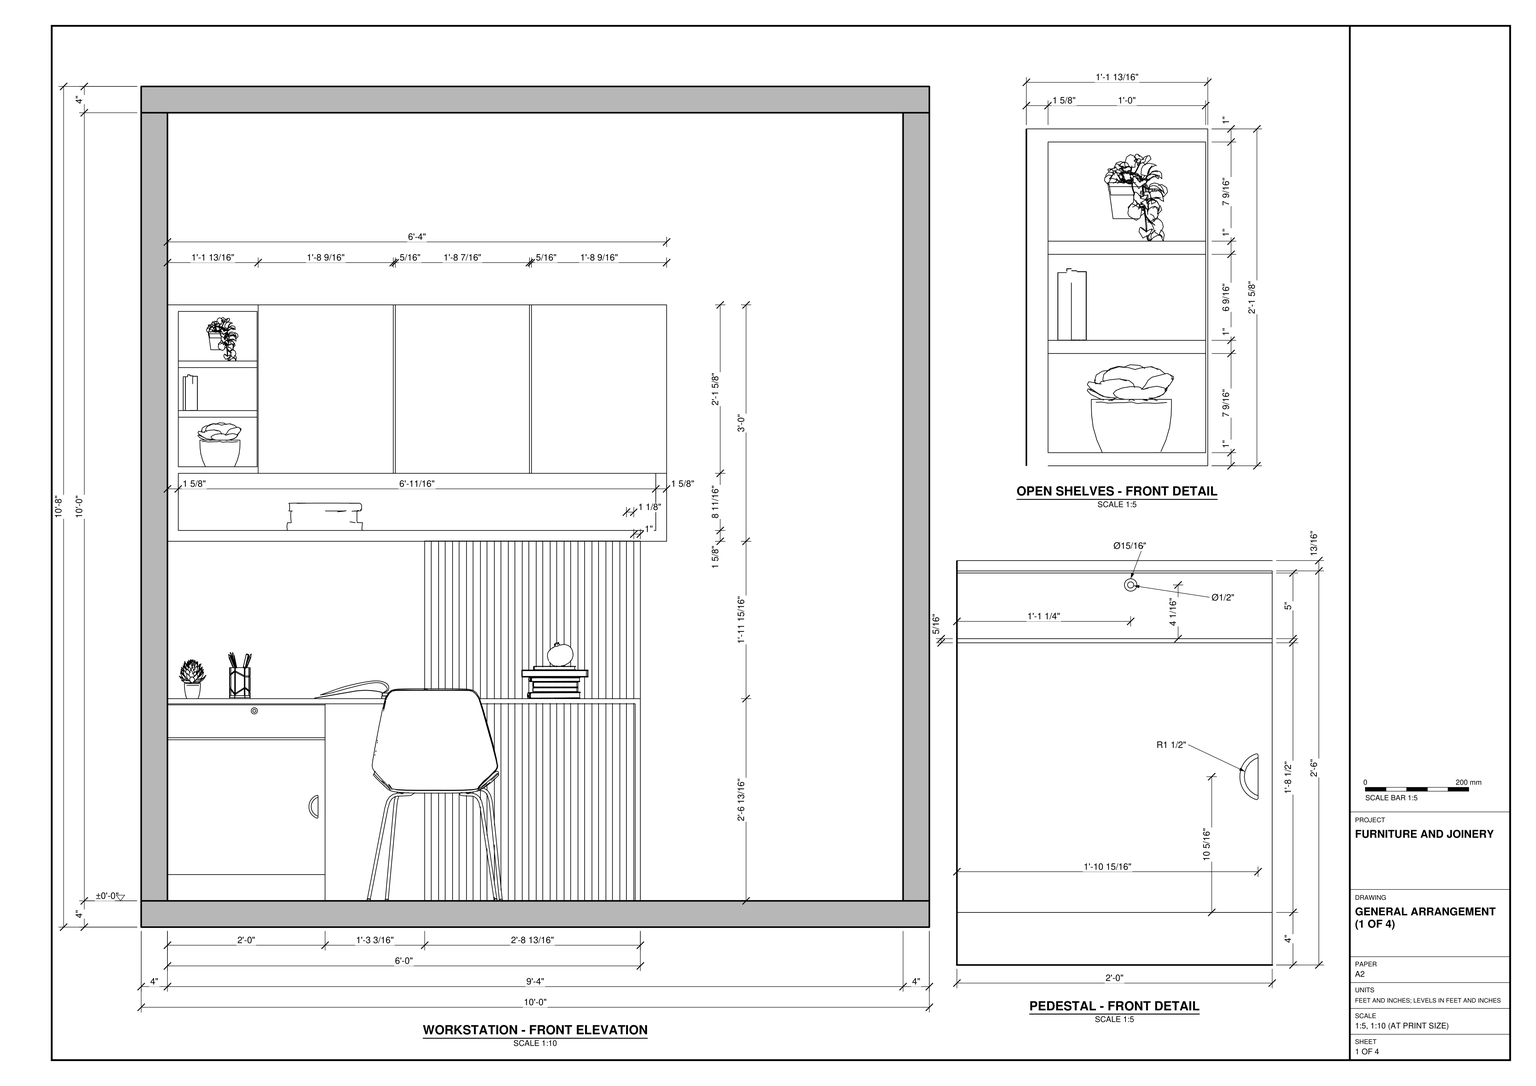
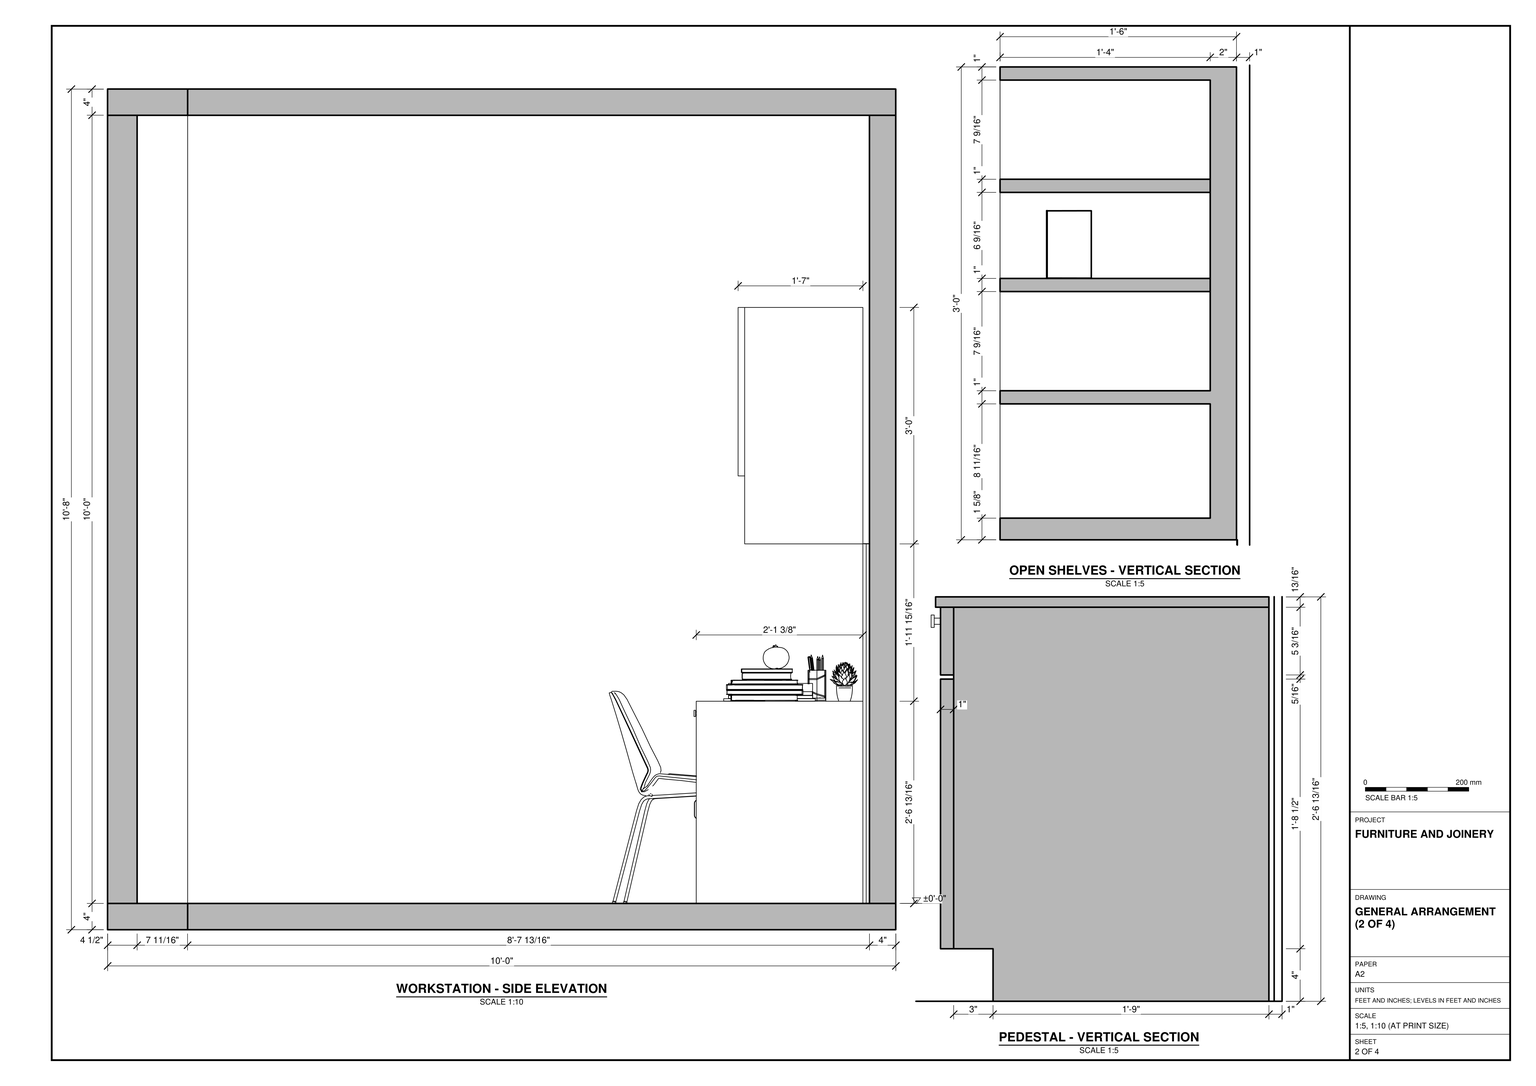
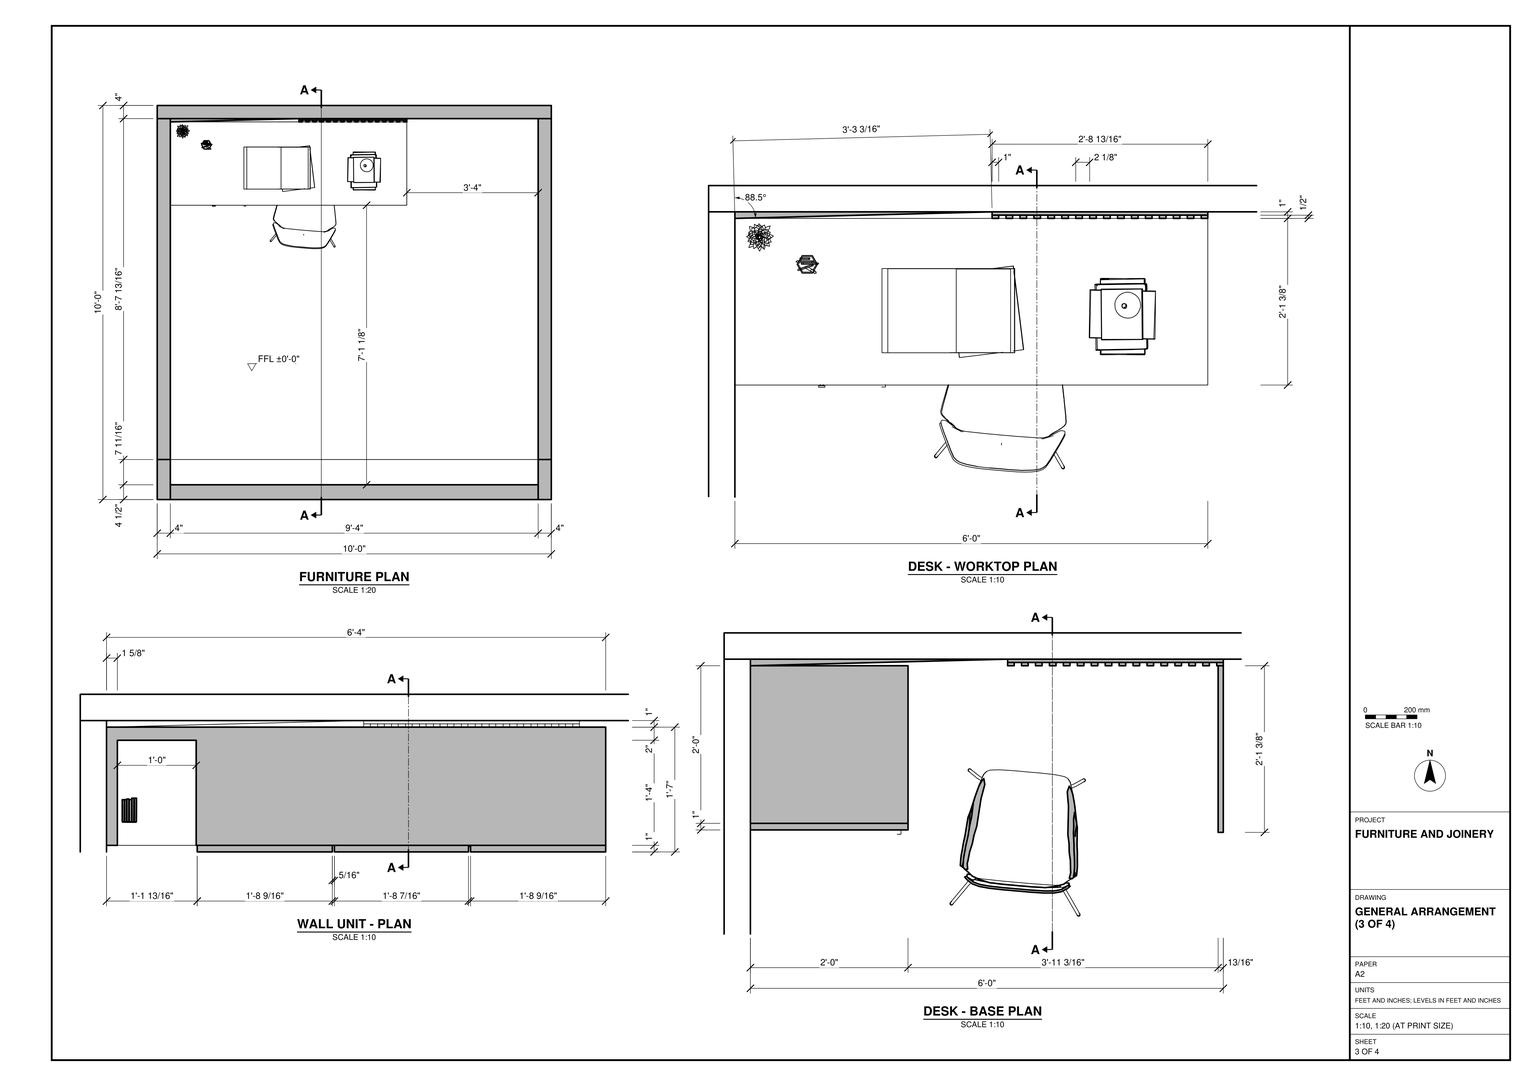
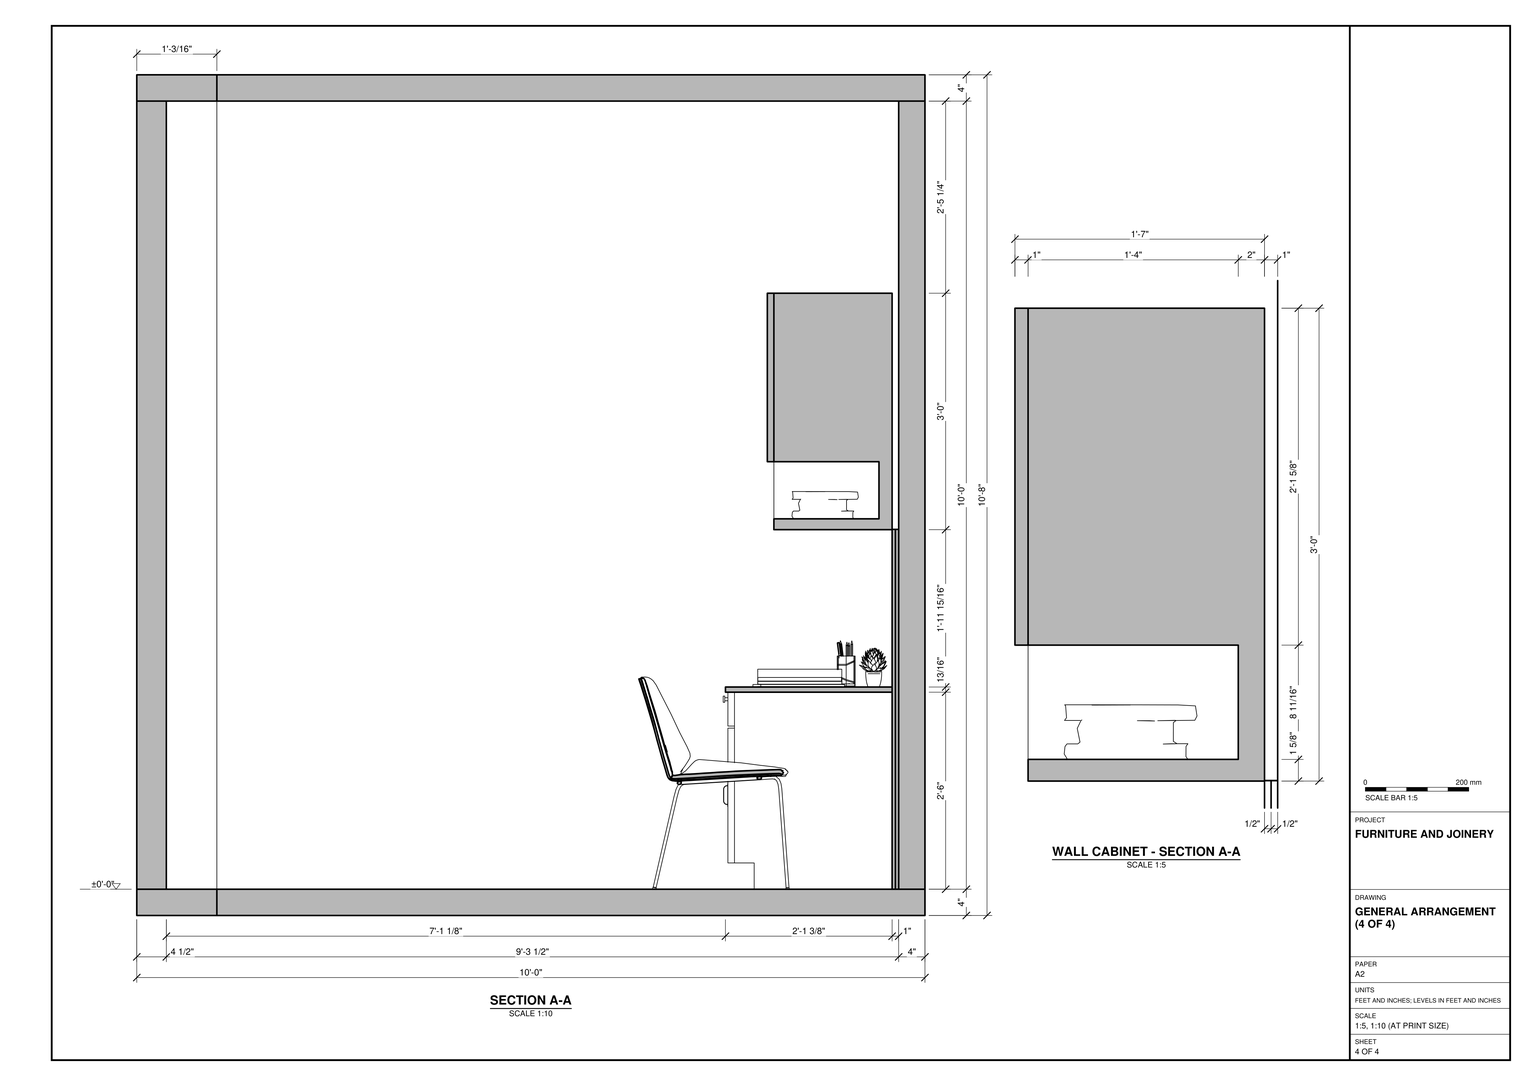
Build the workstation and its room shell in SketchUp from task_files/diagram_01.pdf. Work in feet and inches. The shell measures 10'-0" by 10'-0" in plan and 10'-8" in overall height. Use ±0'-0" as the finished floor level. Follow the wall thicknesses in plan and the floor and ceiling slab thicknesses in elevation.

Fit the desk against the back wall, starting at the left wall and leaving the space shown to its right. Model the continuous worktop, left storage pedestal and thin right end panel. Give the pedestal a shallow drawer above a cupboard door, with the pulls and recessed base shown in the details. Run the vertical slatted backing behind the right portion of the desk, from the floor to the underside of the wall unit. Above the desk, model the narrow stack of open cubbies on the left, the three cabinet fronts to their right and the continuous open shelf below. Place the chair facing the worktop in the knee space.

Decor and loose items such as the plants, books and pencil holders may be any suitable library components. Keep the shell elements and each furniture or joinery piece in separate groups or components, and use components for repeated parts. Save one SketchUp model as output_files/built_in_workstation_with_a_desk_and_wall_storage.skp.

# SketchUp Ruby script. Lengths in inches.
U = 1.inch
M = Sketchup.active_model
def pt(a) = Geom::Point3d.new(a.map { |v| v * U })
def face(e, loops, mat)
  f = e.add_face(loops[0].map { |a| pt(a) })
  loops[1..].each { |l| e.add_face(l.map { |a| pt(a) }).erase! }
  f.material = f.back_material = mat if mat
  f
end
# faces: each face lists its corners as indices into pts; further lists are holes
def faces(e, pts, list, mat = nil) = list.each { |f| face(e, (f[0].is_a?(Array) ? f : [f]).map { |l| l.map { |i| pts[i] } }, mat) }
# xy, xz, yz: faces in a plane at the given z, y or x. An outline is a flat list of corners, or four numbers for a rectangle; further outlines are holes
def ring(l) = l.size == 4 ? [[l[0], l[1]], [l[2], l[1]], [l[2], l[3]], [l[0], l[3]]] : l.each_slice(2).to_a
def flat(e, list, mat, &to3) = list.each { |f| face(e, (f[0].is_a?(Array) ? f : [f]).map { |l| ring(l).map { |u, v| to3.(u, v) } }, mat) }
def xy(e, z, list, mat = nil) = flat(e, list, mat) { |x, y| [x, y, z] }
def xz(e, y, list, mat = nil) = flat(e, list, mat) { |x, z| [x, y, z] }
def yz(e, x, list, mat = nil) = flat(e, list, mat) { |y, z| [x, y, z] }
def lines(e, pts, list) = list.each { |a, b| e.add_line(pt(pts[a]), pt(pts[b])) }
# prism: a flat outline (further loops are holes) pulled along v
def prism(e, loops, v, mat = nil)
  f = face(e, loops, mat); d = Geom::Vector3d.new(v.map { |x| x * U })
  f.pushpull(f.normal.samedirection?(d) ? d.length : -d.length)
end
def box(e, o, s, mat = nil) = prism(e, [[o, [o[0] + s[0], o[1], o[2]], [o[0] + s[0], o[1] + s[1], o[2]], [o[0], o[1] + s[1], o[2]]]], [0, 0, s[2]], mat)
def at(x, y, z, deg = 0) = Geom::Transformation.translation(pt([x, y, z])) * Geom::Transformation.rotation(ORIGIN, Z_AXIS, deg.degrees)
def axes(o, x, y, z) = Geom::Transformation.new([*x, 0, *y, 0, *z, 0, *pt(o).to_a, 1])
def part(name) = M.definitions.add(name)
# library, detail: a bought-in or finely detailed component or shape, given as its bounding box
def library(name, o, s) = part(name).tap { |d| box(d.entities, o, s) }
def detail(e, o, s) = box(e.add_group.entities, o, s)
def put(e, d, t, mat = nil) = e.add_instance(d, t).tap { |i| i.material = mat if mat }
def group(e, t, mat = nil) = e.add_group.tap { |g| g.transformation = t; g.material = mat if mat }.entities
root = M.entities
M.materials.add("Carpaint White 004 1.79cm").color = [255, 255, 255]
M.materials.add("Tiles Simple 01 100cm").color = [188, 184, 182]
M.materials.add("Wall Paint Olive Satin 300cm").color = [133, 140, 86]
M.materials.add("Wood Teak 33-35 100cm\#1").color = [135, 81, 33]
M.materials.add("XPS Yellow SSS 1.51cm").color = [255, 255, 255]
M.materials.add("[Color M09]4").color = [0, 0, 0]
c1 = library("Handle_25.skp\#1",[-1.74,-0.67,0],[3.48,0.67,1.38])
c2 = library("Potted Plant 50-24",[-2.18,-2.1,0],[4.36,4.2,6.7])
c3 = library("Potted Plant 50-23",[-3.4,-3.5,0],[6.8,7,9.93])
c4 = library("Books 53-17",[-2.19,-3.6875,0],[4.38,7.37,10.99])
c5 = library("Books 274 007",[-5.76,-5.0625,0],[11.51,10.11,4.16])
c6 = library("Chair 035",[-9.96,-11.17,0],[19.92,22.29,32.3125])
c7 = library("Plant 260 031 02",[-5.66,-10.61,-5.67],[17.04,23.05,21.91])
c8 = part("Group64\#1")
p = [[0,0,0],[0,0,-12.26],[-5.84,0,-12.26],[38,-1.69,0],[-38,-1.69,0],[38,1.69,0],
  [38,0,0],[-38,1.69,0],[5.84,0,-12.26],[-38,0,0],[0,0,-19.85]]
lines(c8.entities,p,[[0,1],[1,2],[3,4],[5,6],[7,5],[1,8],[9,0],[0,6],[8,10],[4,9],[6,3],[2,10],
  [9,7]])
c9 = part("Rectangle Light")
put(c9.entities,c8,at(0,0,0))
c10 = part("Group\#1")
xy(c10.entities,0,[[0,0,120,120]])
xy(c10.entities,4,[[0,0,120,120]],"Tiles Simple 01 100cm")
xz(c10.entities,0,[[0,0,120,4]])
xz(c10.entities,120,[[0,0,120,4]])
yz(c10.entities,0,[[0,0,120,4]])
yz(c10.entities,120,[[0,0,120,4]])
c11 = part("Group\#12")
box(c11.entities,[0,0,0],[12,16,1])
c12 = part("Group\#27")
box(c12.entities,[0,0,0],[1,0.5,54.79])
c13 = part("Group70\#1")
xz(c13.entities,27.01,[[10.27,0,130.27,4]])
c14 = part("Group74\#1")
xz(c14.entities,27.01,[[10.27,4,14.27,124]])
c15 = part("Group76\#1")
xz(c15.entities,27.01,[[126.27,4,130.27,124]])
c16 = part("Group208\#1")
xz(c16.entities,27.01,[[10.27,124,130.27,128]])
c17 = part("Group67\#1")
put(c17.entities,c13,at(0,0,0))
put(c17.entities,c14,at(0,0,0))
put(c17.entities,c15,at(0,0,0))
put(c17.entities,c16,at(0,0,0))
c18 = library("Group\#30",[0,0,0],[72,25.375,39.39])
put(root,c1,axes([26.93,90,18.33],[0,0,1],[0,1,0],[-1,0,0]))
put(root,c2,axes([11.92,103.93,70.09],[1.5048,0,0],[0,1,0],[0,0,1]))
put(root,c3,axes([7.83,112.1,34.79],[0.6,0,0],[0,0.6,0],[0,0,0.6]))
put(root,c4,axes([7.48,102.36,78.64],[0.4968,0,0],[0,0.4968,0],[0,0,0.4968]))
put(root,c5,at(27.94,104.8125,60.4))
put(root,c6,at(45.14,87.71,4,175))
put(root,c7,axes([11.54,100,87.91],[0.28224,0,0],[0,0.224,0],[0,0,0.3024]))
put(root,c9,axes([42,113.31,58.73],[1,0,0],[0,-1,0],[0,0,0.11]))
put(root,c10,at(0,0,0))
g1 = group(root,at(0,116,4))
xy(g1,0,[[0,0,120,4]])
xy(g1,120,[[0,0,120,4]])
xz(g1,0,[[0,0,120,120]],"Carpaint White 004 1.79cm")
xz(g1,4,[[0,0,120,120]])
yz(g1,0,[[0,0,4,120]])
yz(g1,120,[[0,0,4,120]])
p = [[43.16,0,0],[43.16,0,54.74],[4,-1,54.74],[4,-1,0]]
faces(g1,p,[[0,1,2,3]],"XPS Yellow SSS 1.51cm")
g2 = group(root,at(0,0,4))
xy(g2,0,[[0,0,4,116]])
xy(g2,120,[[0,0,4,116]])
xz(g2,0,[[0,0,4,120]])
xz(g2,116,[[0,0,4,120]])
yz(g2,0,[[0,0,116,120]])
yz(g2,4,[[0,0,116,120]],"Carpaint White 004 1.79cm")
g3 = group(root,at(116,0,4))
box(g3,[0,0,0],[4,116,120])
g4 = group(root,at(4,97,58.74),"Wall Paint Olive Satin 300cm")
xy(g4,0,[[0,0,76,18]])
xy(g4,1.65,[[1.65,0,74.35,16]])
xy(g4,10.35,[[1.65,0,74.35,16]])
xy(g4,11.35,[[1.65,0,13.65,16]])
xy(g4,35,[[1.65,0,13.65,16]])
xy(g4,36,[[0,0,76,18]])
xz(g4,0,[[[0,0,76,36],[1.65,1.65,74.35,10.35],[1.65,11.35,13.65,35]]])
xz(g4,16,[[1.65,1.65,74.35,10.35],[1.65,11.35,13.65,35]])
xz(g4,18,[[0,0,76,36]])
yz(g4,0,[[0,0,18,36]])
yz(g4,1.65,[[0,1.65,16,10.35],[0,11.35,16,35]])
yz(g4,13.65,[[0,11.35,16,35]])
yz(g4,74.35,[[0,1.65,16,10.35]])
yz(g4,76,[[0,0,18,36]])
g5 = group(root,at(17.81,96,69.09),"XPS Yellow SSS 1.51cm")
xy(g5,0,[[0,0,20.57,1],[20.89,0,41.3,1],[41.62,0,62.19,1]])
xy(g5,25.65,[[0,0,20.57,1],[20.89,0,41.3,1],[41.62,0,62.19,1]])
xz(g5,0,[[0,0,20.57,25.65],[20.89,0,41.3,25.65],[41.62,0,62.19,25.65]])
xz(g5,1,[[0,0,20.57,25.65],[20.57,0,20.89,25.65],[20.89,0,41.3,25.65],[41.3,0,41.62,25.65],[41.62,0,62.19,25.65]])
yz(g5,0,[[0,0,1,25.65]])
yz(g5,20.57,[[0,0,1,25.65]])
yz(g5,20.89,[[0,0,1,25.65]])
yz(g5,41.3,[[0,0,1,25.65]])
yz(g5,41.62,[[0,0,1,25.65]])
yz(g5,62.19,[[0,0,1,25.65]])
put(root,c11,at(5.65,97,77.64),"Wall Paint Olive Satin 300cm")
put(root,c11,at(5.65,97,85.19),"Wall Paint Olive Satin 300cm")
g6 = group(root,at(16.75,89.28,32.46))
xz(g6,0,[[0.47,0,0.6,0.02,0.71,0.0625,0.81,0.14,0.89,0.24,0.93,0.35,0.95,0.47,0.93,0.6,0.89,0.71,0.81,0.81,0.71,0.89,0.6,0.93,0.47,0.95,0.35,0.93,0.24,0.89,0.14,0.81,0.0625,0.71,0.02,0.6,0,0.47,0.02,0.35,0.0625,0.24,0.14,0.14,0.24,0.0625,0.35,0.02]],"[Color M09]4")
xz(g6,0.24,[[[0.47,0,0.35,0.02,0.24,0.0625,0.14,0.14,0.0625,0.24,0.02,0.35,0,0.47,0.02,0.6,0.0625,0.71,0.14,0.81,0.24,0.89,0.35,0.93,0.47,0.95,0.6,0.93,0.71,0.89,0.81,0.81,0.89,0.71,0.93,0.6,0.95,0.47,0.93,0.35,0.89,0.24,0.81,0.14,0.71,0.0625,0.6,0.02],[0.47,0.24,0.54,0.25,0.59,0.27,0.64,0.31,0.68,0.36,0.7,0.41,0.71,0.47,0.7,0.54,0.68,0.59,0.64,0.64,0.59,0.68,0.54,0.7,0.47,0.71,0.41,0.7,0.36,0.68,0.31,0.64,0.27,0.59,0.25,0.54,0.24,0.47,0.25,0.41,0.27,0.36,0.31,0.31,0.36,0.27,0.41,0.25]]],"[Color M09]4")
p = [[0.24,0.24,0.0625],[0.35,0.24,0.02],[0.35,0,0.02],[0.24,0,0.0625],[0.47,0.24,0],[0.47,0,0],
  [0.6,0.24,0.02],[0.6,0,0.02],[0.71,0.24,0.0625],[0.71,0,0.0625],[0.14,0.24,0.14],[0.14,0,0.14],
  [0.0625,0.24,0.24],[0.0625,0,0.24],[0.81,0.24,0.14],[0.81,0,0.14],[0.89,0.24,0.24],[0.89,0,0.24],
  [0.02,0.24,0.35],[0.02,0,0.35],[0.93,0.24,0.35],[0.93,0,0.35],[0.41,0.71,0.25],[0.47,0.71,0.24],
  [0.47,0.24,0.24],[0.41,0.24,0.25],[0.36,0.71,0.27],[0.36,0.24,0.27],[0.54,0.71,0.25],[0.54,0.24,0.25],
  [0.59,0.71,0.27],[0.59,0.24,0.27],[0.27,0.71,0.36],[0.31,0.71,0.31],[0.31,0.24,0.31],[0.27,0.24,0.36],
  [0.64,0.71,0.31],[0.64,0.24,0.31],[0.68,0.71,0.36],[0.68,0.24,0.36],[0,0.24,0.47],[0,0,0.47],
  [0.95,0.24,0.47],[0.95,0,0.47],[0.24,0.71,0.47],[0.25,0.71,0.41],[0.25,0.24,0.41],[0.24,0.24,0.47],
  [0.7,0.71,0.41],[0.71,0.71,0.47],[0.71,0.24,0.47],[0.7,0.24,0.41],[0.02,0.24,0.6],[0.02,0,0.6],
  [0.93,0.24,0.6],[0.93,0,0.6],[0.25,0.71,0.54],[0.25,0.24,0.54],[0.27,0.71,0.59],[0.27,0.24,0.59],
  [0.7,0.71,0.54],[0.7,0.24,0.54],[0.68,0.71,0.59],[0.68,0.24,0.59],[0.0625,0.24,0.71],[0.0625,0,0.71],
  [0.89,0.24,0.71],[0.89,0,0.71],[0.36,0.71,0.68],[0.31,0.71,0.64],[0.31,0.24,0.64],[0.36,0.24,0.68],
  [0.64,0.71,0.64],[0.59,0.71,0.68],[0.59,0.24,0.68],[0.64,0.24,0.64],[0.14,0.24,0.81],[0.14,0,0.81],
  [0.81,0.24,0.81],[0.81,0,0.81],[0.41,0.71,0.7],[0.41,0.24,0.7],[0.47,0.71,0.71],[0.47,0.24,0.71],
  [0.54,0.71,0.7],[0.54,0.24,0.7],[0.24,0.24,0.89],[0.24,0,0.89],[0.71,0.24,0.89],[0.71,0,0.89],
  [0.35,0.24,0.93],[0.35,0,0.93],[0.47,0.24,0.95],[0.47,0,0.95],[0.6,0.24,0.93],[0.6,0,0.93]]
faces(g6,p,[[0,1,2,3],[1,4,5,2],[4,6,7,5],[6,8,9,7],[10,0,3,11],[12,10,11,13],[8,14,15,9],[14,16,17,15],
  [18,12,13,19],[16,20,21,17],[22,23,24,25],[26,22,25,27],[23,28,29,24],[28,30,31,29],[32,33,34,35],[33,26,27,34],
  [30,36,37,31],[36,38,39,37],[40,18,19,41],[20,42,43,21],[44,45,46,47],[45,32,35,46],[48,49,50,51],[38,48,51,39],
  [52,40,41,53],[42,54,55,43],[56,44,47,57],[58,56,57,59],[49,60,61,50],[60,62,63,61],[64,52,53,65],[54,66,67,55],
  [68,69,70,71],[69,58,59,70],[72,73,74,75],[62,72,75,63],[76,64,65,77],[66,78,79,67],[80,68,71,81],[82,80,81,83],
  [84,82,83,85],[73,84,85,74],[86,76,77,87],[78,88,89,79],[90,86,87,91],[92,90,91,93],[94,92,93,95],[88,94,95,89]],"[Color M09]4")
g7 = group(root,at(43.16,115,4),"Wood Teak 33-35 100cm\#1")
g8 = group(g7,at(0,0.5,0))
box(g8,[0,0,0],[32.84,0.5,54.79])
g9 = group(g7,at(0,0,0))
box(g9,[0,0,0],[1,0.5,54.79])
put(g7,c12,at(2.12,0,0))
put(g7,c12,at(4.25,0,0))
put(g7,c12,at(6.37,0,0))
put(g7,c12,at(21.23,0,0))
put(g7,c12,at(23.35,0,0))
put(g7,c12,at(14.86,0,0))
put(g7,c12,at(27.59,0,0))
put(g7,c12,at(29.72,0,0))
put(g7,c12,at(31.84,0,0))
put(g7,c12,at(8.49,0,0))
put(g7,c12,at(16.98,0,0))
put(g7,c12,at(25.47,0,0))
g10 = group(g7,at(10.61,0,0))
box(g10,[0,0,0],[1,0.5,54.79])
put(g7,c12,at(12.74,0,0))
put(g7,c12,at(19.1,0,0))
g11 = group(root,at(4,0,4))
box(g11,[0,0,0],[112,4.5,120])
put(root,c10,at(0,0,124))
put(root,c17,at(-10.27,-14.82,0))
put(root,c18,at(4,89.625,4))
